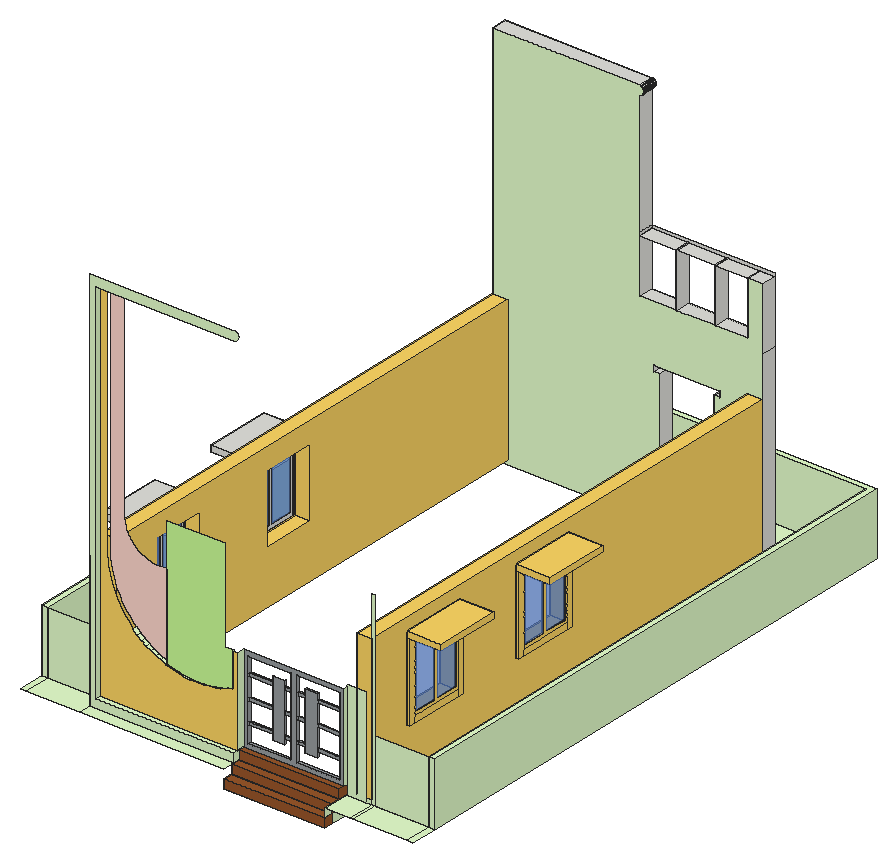
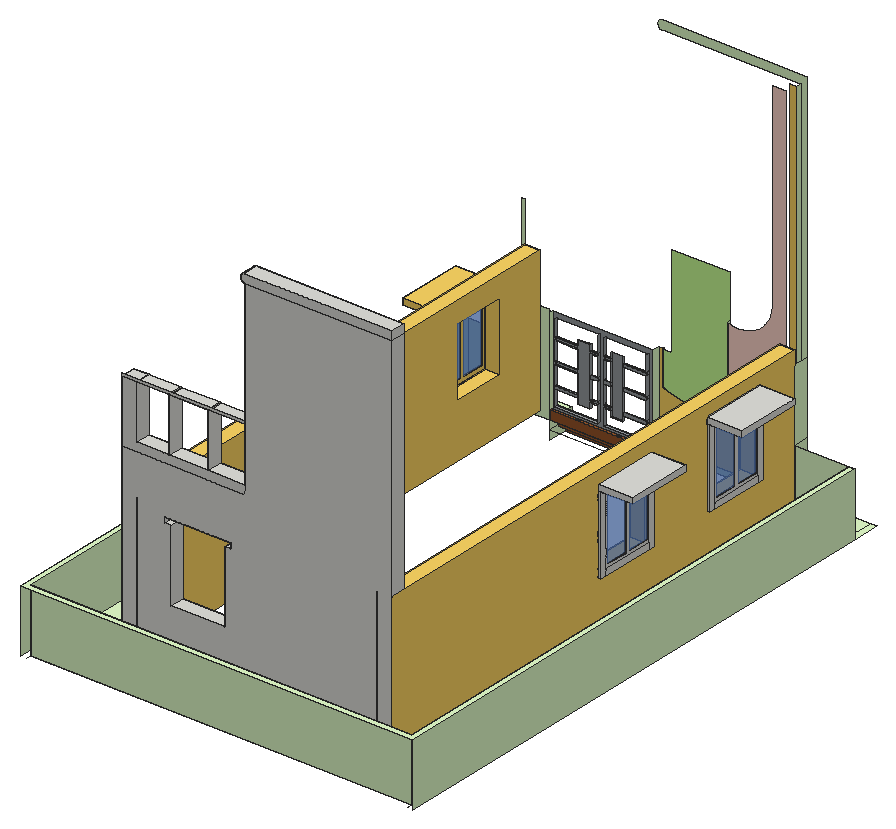
# SketchUp Ruby script. Lengths in inches.
U = 1.inch
M = Sketchup.active_model
def pt(a) = Geom::Point3d.new(a.map { |v| v * U })
def face(e, loops, mat)
  f = e.add_face(loops[0].map { |a| pt(a) })
  loops[1..].each { |l| e.add_face(l.map { |a| pt(a) }).erase! }
  f.material = f.back_material = mat if mat
  f
end
# faces: each face lists its corners as indices into pts; further lists are holes
def faces(e, pts, list, mat = nil) = list.each { |f| face(e, (f[0].is_a?(Array) ? f : [f]).map { |l| l.map { |i| pts[i] } }, mat) }
# xy, xz, yz: faces in a plane at the given z, y or x. An outline is a flat list of corners, or four numbers for a rectangle; further outlines are holes
def ring(l) = l.size == 4 ? [[l[0], l[1]], [l[2], l[1]], [l[2], l[3]], [l[0], l[3]]] : l.each_slice(2).to_a
def flat(e, list, mat, &to3) = list.each { |f| face(e, (f[0].is_a?(Array) ? f : [f]).map { |l| ring(l).map { |u, v| to3.(u, v) } }, mat) }
def xy(e, z, list, mat = nil) = flat(e, list, mat) { |x, y| [x, y, z] }
def xz(e, y, list, mat = nil) = flat(e, list, mat) { |x, z| [x, y, z] }
def yz(e, x, list, mat = nil) = flat(e, list, mat) { |y, z| [x, y, z] }
def lines(e, pts, list) = list.each { |a, b| e.add_line(pt(pts[a]), pt(pts[b])) }
# prism: a flat outline (further loops are holes) pulled along v
def prism(e, loops, v, mat = nil)
  f = face(e, loops, mat); d = Geom::Vector3d.new(v.map { |x| x * U })
  f.pushpull(f.normal.samedirection?(d) ? d.length : -d.length)
end
def box(e, o, s, mat = nil) = prism(e, [[o, [o[0] + s[0], o[1], o[2]], [o[0] + s[0], o[1] + s[1], o[2]], [o[0], o[1] + s[1], o[2]]]], [0, 0, s[2]], mat)
def at(x, y, z, deg = 0) = Geom::Transformation.translation(pt([x, y, z])) * Geom::Transformation.rotation(ORIGIN, Z_AXIS, deg.degrees)
def axes(o, x, y, z) = Geom::Transformation.new([*x, 0, *y, 0, *z, 0, *pt(o).to_a, 1])
def part(name) = M.definitions.add(name)
# library, detail: a bought-in or finely detailed component or shape, given as its bounding box
def library(name, o, s) = part(name).tap { |d| box(d.entities, o, s) }
def detail(e, o, s) = box(e.add_group.entities, o, s)
def put(e, d, t, mat = nil) = e.add_instance(d, t).tap { |i| i.material = mat if mat }
def group(e, t, mat = nil) = e.add_group.tap { |g| g.transformation = t; g.material = mat if mat }.entities
root = M.entities
M.materials.add("[Color B01]").color = [255, 216, 204]
M.materials.add("[Color D03]").color = [255, 216, 101]
M.materials.add("[Color F01]").color = [229, 255, 204]
M.materials.add("[Color F02]").color = [204, 255, 153]
M.materials.add("[Metal Rough]").color = [153, 157, 160]
M.materials.add("[Translucent Glass Blue]").color = [100, 149, 237]
M.materials["[Translucent Glass Blue]"].alpha = 0.5
M.materials.add("[Wood Cherry Original]").color = [152, 86, 42]
c1 = part("Group\#15")
box(c1.entities,[0,0,0],[67,6,6])
c2 = part("Difference\#2")
prism(c2.entities,[[[10,0,96],[10,0,0],[10,336,0],[10,336,96]],[[10,69,82],[10,69,36],[10,33,36],[10,33,82]],[[10,125,36],[10,125,82],[10,161,82],[10,161,36]]],[-10,0,0])
c3 = part("Group\#28")
box(c3.entities,[0,0,0],[0.5,16,22])
c4 = part("Group\#37")
yz(c4.entities,23,[[0,0,4,28],[4,0,40,4]])
p = [[23,40,28],[23,44,28],[23,40,4]]
lines(c4.entities,p,[[0,1],[0,2]])
g1 = group(c4.entities,at(23,4,0))
xz(g1,0,[[-2,0,0,4]])
g2 = group(g1,at(0,0,0))
xy(g2,0,[[-2,0,0,36]])
xy(g2,4,[[-2,0,0,36]])
xz(g2,36,[[-2,0,0,4]])
yz(g2,-2,[[0,0,36,4]])
yz(g2,0,[[0,0,36,4]])
g3 = group(c4.entities,at(23,40,0))
box(g3,[-2,0,0],[2,4,52])
g4 = group(c4.entities,at(23,0,0))
box(g4,[-2,0,0],[2,4,52])
g5 = group(c4.entities,at(22,4,4))
prism(g5,[[[0,0,0],[0,0,48],[0,36,48],[0,36,0]],[[0,35,46],[0,19,46],[0,19,2],[0,35,2]],[[0,1,2],[0,17,2],[0,17,46],[0,1,46]]],[-1,0,0])
put(g5,c3,axes([0,19,2],[-1,0,0],[0,1,0],[0,0,2]),"[Translucent Glass Blue]")
put(g5,c3,axes([-0.23,1,2],[-1,0,0],[0,1,0],[0,0,2]),"[Translucent Glass Blue]")
g6 = group(c4.entities,at(0,0,52))
yz(g6,23,[[0,0,44,4]])
g7 = group(g6,at(0,0,0))
xy(g7,0,[[0,0,23,44]])
xy(g7,4,[[0,0,23,44]])
xz(g7,0,[[0,0,23,4]])
xz(g7,44,[[0,0,23,4]])
yz(g7,0,[[0,0,44,4]])
xy(root,21,[[0,344.07,4,362.07],[4,344.07,40,362.07],[40,344.07,136,352.07],[203,344.07,220,362.07],[220,344.07,222,362.07],
  [222,344.07,258,362.07],[258,344.07,262,362.07],[4,362.07,40,362.07,40,698.07,220,698.07,220,362.07,258,362.07,258,726.37,4,726.37]],"[Color F01]")
xy(root,27,[[44,352.07,136,355.07],[136,360.07,203,362.07]],"[Color F01]")
xy(root,30,[[139,360.07,167.5,362.07],[171.5,360.07,200,362.07]],"[Metal Rough]")
xy(root,37.02,[[154.51,361.07,162.66,362.07],[176.34,361.07,184.49,362.07]],"[Metal Rough]")
xy(root,40.7,[[139,361.07,154.51,362.07],[162.66,361.07,167.5,362.07],[171.5,361.07,176.34,362.07],[184.49,361.07,200,362.07]],"[Metal Rough]")
xy(root,42.7,[[139,361.07,154.51,362.07],[162.66,361.07,167.5,362.07],[171.5,361.07,176.34,362.07],[184.49,361.07,200,362.07]],"[Metal Rough]")
xy(root,55.2,[[139,361.07,154.51,362.07],[162.66,361.07,167.5,362.07],[171.5,361.07,176.34,362.07],[184.49,361.07,200,362.07]],"[Metal Rough]")
xy(root,57.2,[[139,361.07,154.51,362.07],[162.66,361.07,167.5,362.07],[171.5,361.07,176.34,362.07],[184.49,361.07,200,362.07]],"[Metal Rough]")
xy(root,63,[[0,362.07,4,362.07,4,726.37,258,726.37,258,362.07,262,362.07,262,730.07,0,730.07]],"[Color F01]")
xy(root,69.7,[[139,361.07,154.51,362.07],[162.66,361.07,167.5,362.07],[171.5,361.07,176.34,362.07],[184.49,361.07,200,362.07]],"[Metal Rough]")
xy(root,71.7,[[139,361.07,154.51,362.07],[162.66,361.07,167.5,362.07],[171.5,361.07,176.34,362.07],[184.49,361.07,200,362.07]],"[Metal Rough]")
xz(root,352.07,[[40,21,136,21,136,27,44,27,44,273,136,273,136.38,273.02,136.76,273.1,136.95,273.15,137.125,273.22,137.3,273.3,137.47,273.39,137.64,273.49,137.79,273.6,138.09,273.84,138.22,273.98,138.35,274.13,138.46,274.28,138.57,274.44,138.66,274.61,138.74,274.79,138.82,274.96,138.875,275.15,138.92,275.33,138.96,275.52,138.99,275.71,139,275.9,139,276.1,138.99,276.29,138.96,276.48,138.92,276.67,138.875,276.85,138.82,277.04,138.74,277.21,138.66,277.39,138.57,277.56,138.46,277.72,138.35,277.87,138.22,278.02,138.09,278.16,137.79,278.4,137.64,278.51,137.47,278.61,137.3,278.7,137.125,278.78,136.95,278.85,136.76,278.9,136.38,278.98,136,279,40,279]],"[Color F01]")
xz(root,355.07,[[44,27,136,27,136,85.4,133,85.4,133,62.89,129.08,61.43,125.07,60.24,121,59.31,116.87,58.64,112.71,58.24,108.53,58.11,104.36,58.26,100.2,58.67,96.07,59.36,92,60.3,88,61.51,84.6,62.85,81.28,64.39,78.07,66.14,74.97,68.08,72,70.21,69.17,72.52,66.49,75.01,63.97,77.66,61.61,80.45,59.44,83.39,58.14,85.4,57.45,86.46,55.66,89.65,54.07,92.9375,52.6875,96.32,51.52,99.79,50.57,103.32,49.84,106.9,49.33,110.52,49.05,114.16,49,117.82,49,273,44,273]],"[Color D03]")
xz(root,356.07,[[108.53,58.11,112.71,58.24,116.87,58.64,121,59.31,125.07,60.24,129.08,61.43,133,62.89,133,85.4,126.51,85.4,126.51,147,88,147,88,61.51,92,60.3,96.07,59.36,100.2,58.67,104.36,58.26]],"[Color F02]")
xz(root,358.07,[[88,61.51,88,117.88,86.6,117.45,85.18,117.1,83.75,116.85,82.29,116.69,80.83,116.63,79.37,116.66,77.92,116.78,76.47,117,75.04,117.3125,73.64,117.71,72.26,118.2,70.92,118.78,69.62,119.45,68.36,120.19,67.16,121.02,66.01,121.92,64.92,122.9,63.9,123.9375,62.94,125.04,62.06,126.21,61.61,126.88,61.25,127.43,60.53,128.7,59.89,130.01,59.33,131.36,58.87,132.75,58.49,134.16,58.2,135.59,58.01,137.04,57.91,138.5,57.91,139.96,58,141.42,58,270,49,270,49,117.82,49.05,114.16,49.33,110.52,49.84,106.9,50.57,103.32,51.52,99.79,52.6875,96.32,54.07,92.9375,55.66,89.65,57.45,86.46,58.14,85.4,59.44,83.39,61.61,80.45,63.97,77.66,66.49,75.01,69.17,72.52,72,70.21,74.97,68.08,78.07,66.14,81.28,64.39,84.6,62.85]],"[Color B01]")
xz(root,360.07,[[[136,27,203,85.4],[171.5,30,200,82.4],[139,30,167.5,82.4]]],"[Metal Rough]")
xz(root,361.07,[[154.51,37.02,162.66,75.22],[176.34,37.02,184.49,75.22],[139,40.7,154.51,42.7],[162.66,40.7,167.5,42.7],[171.5,40.7,176.34,42.7],
  [184.49,40.7,200,42.7],[139,55.2,154.51,57.2],[162.66,55.2,167.5,57.2],[171.5,55.2,176.34,57.2],[184.49,55.2,200,57.2],
  [139,69.7,154.51,71.7],[162.66,69.7,167.5,71.7],[171.5,69.7,176.34,71.7],[184.49,69.7,200,71.7]],"[Metal Rough]")
xz(root,362.07,[[0,21,4,63],[4,21,40,63],[203,21,216,21,216,87,204.57,87,204.33,86.94,204.21,86.9,204.09,86.85,203.87,86.73,203.77,86.66,203.67,86.58,203.4,86.31,203.33,86.21,203.26,86.1,203.14,85.88,203.02,85.52,203,85.4],[216,21,220,21,220,91.16,219.96,90.87,219.91,90.58,219.83,90.29,219.74,90.01,219.63,89.73,219.5,89.46,219.36,89.2,219.2,88.95,219.02,88.72,218.83,88.49,218.625,88.27,218.41,88.07,218.18,87.89,217.93,87.72,217.68,87.5625,217.42,87.42,217.14,87.3,216.87,87.2,216.58,87.11,216.29,87.05,216,87],[220,21,222,147],
  [222,21,258,63],[258,21,262,63]],"[Color F01]")
xz(root,362.07,[[176.34,37.02,184.49,75.22],[139,40.7,154.51,42.7],[184.49,40.7,200,42.7],[139,55.2,154.51,57.2],[162.66,55.2,167.5,57.2],
  [171.5,55.2,176.34,57.2],[139,69.7,154.51,71.7]],"[Metal Rough]")
xz(root,688.07,[[[40,21,220,21,220,189,210,189,210,153,188.6,153,188.6,189,187.6,189,187.6,153,162.6,153,162.6,189,161.6,189,161.6,153,137.6,153,137.6,273,138.375,273.1,139.1,273.4,139.72,273.88,140.19,274.5,140.49,275.22,140.59,276,140.49,276.77,140.19,277.5,139.72,278.12,139.1,278.59,138.375,278.89,137.6,278.99,137.6,279,40,279],[151.19,63,151.19,111,147.19,111,147.19,115,191.19,115,191.19,111,187.19,111,187.19,63]]],"[Color F01]")
xz(root,726.37,[[4,21,258,63]],"[Color F01]")
yz(root,0,[[362.07,21,730.07,63]],"[Color F01]")
yz(root,4,[[362.07,21,726.37,63]],"[Color F01]")
yz(root,40,[[352.07,21,362.07,63],[352.07,63,362.07,111]],"[Color F01]")
yz(root,44,[[352.07,27,355.07,273]],"[Color F01]")
yz(root,88,[[356.07,61.51,358.07,117.88]],"[Color F01]")
yz(root,133,[[355.07,62.89,356.07,85.4]],"[Color F01]")
yz(root,136,[[352.07,21,362.07,27],[355.07,27,360.07,85.4]],"[Color F01]")
yz(root,139,[[360.07,30,362.07,40.7],[360.07,40.7,361.07,42.7],[360.07,42.7,362.07,55.2],[360.07,55.2,361.07,57.2],[360.07,57.2,362.07,69.7],
  [360.07,69.7,361.07,71.7],[360.07,71.7,362.07,82.4]],"[Metal Rough]")
yz(root,154.51,[[361.07,37.02,362.07,40.7],[361.07,40.7,362.07,42.7],[361.07,42.7,362.07,55.2],[361.07,55.2,362.07,57.2],[361.07,57.2,362.07,69.7],
  [361.07,69.7,362.07,71.7],[361.07,71.7,362.07,75.22]],"[Metal Rough]")
yz(root,162.66,[[361.07,37.02,362.07,40.7],[361.07,40.7,362.07,42.7],[361.07,42.7,362.07,55.2],[361.07,55.2,362.07,57.2],[361.07,57.2,362.07,69.7],
  [361.07,69.7,362.07,71.7],[361.07,71.7,362.07,75.22]],"[Metal Rough]")
yz(root,167.5,[[360.07,30,362.07,40.7],[360.07,40.7,361.07,42.7],[360.07,42.7,362.07,55.2],[360.07,55.2,361.07,57.2],[360.07,57.2,362.07,69.7],
  [360.07,69.7,361.07,71.7],[360.07,71.7,362.07,82.4]],"[Metal Rough]")
yz(root,171.5,[[360.07,30,362.07,40.7],[360.07,40.7,361.07,42.7],[360.07,42.7,362.07,55.2],[360.07,55.2,361.07,57.2],[360.07,57.2,362.07,57.2,362.07,69.7,361.07,69.7,361.07,71.7,360.07,71.7],
  [360.07,71.7,362.07,82.4]],"[Metal Rough]")
yz(root,176.34,[[361.07,37.02,362.07,40.7],[361.07,42.7,362.07,55.2],[361.07,55.2,362.07,57.2],[361.07,57.2,362.07,69.7],[361.07,71.7,362.07,75.22]],"[Metal Rough]")
yz(root,184.49,[[361.07,37.02,362.07,40.7],[361.07,40.7,362.07,42.7],[361.07,42.7,362.07,55.2],[361.07,57.2,362.07,69.7],[361.07,71.7,362.07,75.22]],"[Metal Rough]")
yz(root,200,[[360.07,30,362.07,40.7],[360.07,40.7,361.07,42.7],[360.07,42.7,362.07,55.2],[360.07,55.2,361.07,57.2],[360.07,57.2,362.07,69.7],
  [360.07,69.7,361.07,71.7],[360.07,71.7,362.07,82.4]],"[Metal Rough]")
yz(root,203,[[344.07,9,362.07,15],[344.07,15,362.07,21],[360.07,27,362.07,85.4]],"[Color F01]")
yz(root,258,[[362.07,21,726.37,63]],"[Color F01]")
yz(root,262,[[362.07,21,730.07,63]],"[Color F01]")
p = [[108.53,355.07,58.11],[108.53,356.07,58.11],[104.36,356.07,58.26],[104.36,355.07,58.26],[112.71,355.07,58.24],[112.71,356.07,58.24],
  [116.87,355.07,58.64],[116.87,356.07,58.64],[100.2,356.07,58.67],[100.2,355.07,58.67],[121,355.07,59.31],[121,356.07,59.31],
  [96.07,356.07,59.36],[96.07,355.07,59.36],[125.07,355.07,60.24],[125.07,356.07,60.24],[92,356.07,60.3],[92,355.07,60.3],
  [129.08,355.07,61.43],[129.08,356.07,61.43],[88,356.07,61.51],[88,355.07,61.51],[133,355.07,62.89],[133,356.07,62.89],
  [88,358.07,61.51],[84.6,358.07,62.85],[84.6,355.07,62.85],[81.28,358.07,64.39],[81.28,355.07,64.39],[78.07,358.07,66.14],
  [78.07,355.07,66.14],[74.97,358.07,68.08],[74.97,355.07,68.08],[72,358.07,70.21],[72,355.07,70.21],[69.17,358.07,72.52],
  [69.17,355.07,72.52],[66.49,358.07,75.01],[66.49,355.07,75.01],[220,698.07,21],[220,698.07,120],[136,362.07,21],
  [203,362.07,21],[136,362.07,15],[203,362.07,15],[258,726.37,21],[258,730.07,21],[4,726.37,21],
  [4,730.07,21]]
faces(root,p,[[0,1,2,3],[4,5,1,0],[6,7,5,4],[3,2,8,9],[10,11,7,6],[9,8,12,13],[14,15,11,10],[13,12,16,17],
  [18,19,15,14],[17,16,20,21],[22,23,19,18],[24,25,26,21,20],[25,27,28,26],[27,29,30,28],[29,31,32,30],[31,33,34,32],
  [33,35,36,34],[35,37,38,36]],"[Color F01]")
lines(root,p,[[39,40],[41,42],[43,44],[45,46],[47,48]])
put(root,c1,axes([136,350.07,9],[1,0,0],[0,0,1],[0,-1,0]),"[Wood Cherry Original]")
put(root,c1,axes([136,356.07,15],[1,0,0],[0,0,1],[0,-1,0]),"[Wood Cherry Original]")
put(root,c1,axes([136,362.07,21],[1,0,0],[0,0,1],[0,-1,0]),"[Wood Cherry Original]")
g8 = group(root,at(220,688.07,21))
xy(g8,168,[[-82.4,0,-58.4,10],[-57.4,0,-32.4,10],[-31.4,0,0,10]])
xz(g8,10,[[-58.4,132,-57.4,168],[-32.4,132,-31.4,168],[-82.4,168,0,170]])
yz(g8,-58.4,[[0,132,10,168]])
yz(g8,-57.4,[[0,132,10,168]])
yz(g8,-32.4,[[0,132,10,168]])
yz(g8,-31.4,[[0,132,10,168]])
g9 = group(g8,at(0,0,0))
xy(g9,0,[[-180,0,0,10]])
xy(g9,42,[[-68.81,0,-32.81,10]])
xy(g9,90,[[-72.81,0,-68.81,10],[-32.81,0,-28.81,10]])
xy(g9,94,[[-72.81,0,-28.81,10]])
xy(g9,132,[[-82.4,0,-58.4,10],[-58.4,0,-57.4,10],[-57.4,0,-32.4,10],[-32.4,0,-31.4,10],[-31.4,0,-10,10]])
xy(g9,168,[[-10,0,0,10]])
xy(g9,258,[[-180,0,-82.4,10]])
xz(g9,10,[[-180,0,0,6],[[-180,6,-180,252,-82.4,252,-82.4,126,0,126,0,6],[-68.81,42,-32.81,42,-32.81,90,-28.81,90,-28.81,94,-72.81,94,-72.81,90,-68.81,90]],[-82.4,126,-82.4,132,-10,132,-10,168,0,168,0,126],[-180,252,-180,258,-82.4,258,-82.02,257.98,-81.64,257.9,-81.46,257.85,-81.28,257.78,-81.1,257.7,-80.93,257.61,-80.77,257.51,-80.61,257.4,-80.46,257.28,-80.32,257.16,-80.18,257.02,-79.94,256.72,-79.84,256.56,-79.74,256.39,-79.66,256.21,-79.59,256.04,-79.53,255.85,-79.48,255.67,-79.44,255.48,-79.4,255.1,-79.4,254.9,-79.44,254.52,-79.48,254.33,-79.53,254.15,-79.59,253.96,-79.66,253.79,-79.74,253.61,-79.84,253.44,-79.94,253.28,-80.18,252.98,-80.32,252.84,-80.46,252.72,-80.61,252.6,-80.77,252.49,-80.93,252.39,-81.1,252.3,-81.28,252.22,-81.46,252.15,-81.64,252.1,-82.02,252.02,-82.4,252]])
yz(g9,-180,[[0,0,10,6],[0,6,10,252],[0,252,10,258]])
yz(g9,-82.4,[[0,132,10,168],[0,168,10,170],[0,170,10,252]])
yz(g9,-79.4,[[0,254.9,10,255.1]])
yz(g9,-72.81,[[0,90,10,94]])
yz(g9,-68.81,[[0,42,10,90]])
yz(g9,-32.81,[[0,42,10,90]])
yz(g9,-28.81,[[0,90,10,94]])
yz(g9,-10,[[0,132,10,168]])
yz(g9,0,[[0,0,10,6],[0,6,10,126],[0,126,10,168]])
p = [[-82.21,0,252.01],[-82.4,0,252],[-82.4,10,252],[-82.21,10,252.01],[-82.02,0,252.02],[-82.02,10,252.02],
  [-81.83,0,252.06],[-81.83,10,252.06],[-81.64,0,252.1],[-81.64,10,252.1],[-81.46,0,252.15],[-81.46,10,252.15],
  [-81.28,0,252.22],[-81.28,10,252.22],[-81.1,0,252.3],[-81.1,10,252.3],[-80.93,0,252.39],[-80.93,10,252.39],
  [-80.77,0,252.49],[-80.77,10,252.49],[-80.61,0,252.6],[-80.61,10,252.6],[-80.46,0,252.72],[-80.46,10,252.72],
  [-80.32,0,252.84],[-80.32,10,252.84],[-80.18,0,252.98],[-80.18,10,252.98],[-80.06,0,253.13],[-80.06,10,253.13],
  [-79.94,0,253.28],[-79.94,10,253.28],[-79.84,0,253.44],[-79.84,10,253.44],[-79.74,0,253.61],[-79.74,10,253.61],
  [-79.66,0,253.79],[-79.66,10,253.79],[-79.59,0,253.96],[-79.59,10,253.96],[-79.53,0,254.15],[-79.53,10,254.15],
  [-79.48,0,254.33],[-79.48,10,254.33],[-79.44,0,254.52],[-79.44,10,254.52],[-79.42,0,254.71],[-79.42,10,254.71],
  [-79.4,0,254.9],[-79.4,10,254.9],[-79.42,0,255.29],[-79.4,0,255.1],[-79.4,10,255.1],[-79.42,10,255.29],
  [-79.44,0,255.48],[-79.44,10,255.48],[-79.48,0,255.67],[-79.48,10,255.67],[-79.53,0,255.85],[-79.53,10,255.85],
  [-79.59,0,256.04],[-79.59,10,256.04],[-79.66,0,256.21],[-79.66,10,256.21],[-79.74,0,256.39],[-79.74,10,256.39],
  [-79.84,0,256.56],[-79.84,10,256.56],[-79.94,0,256.72],[-79.94,10,256.72],[-80.06,0,256.87],[-80.06,10,256.87],
  [-80.18,0,257.02],[-80.18,10,257.02],[-80.32,0,257.16],[-80.32,10,257.16],[-80.46,0,257.28],[-80.46,10,257.28],
  [-80.61,0,257.4],[-80.61,10,257.4],[-80.77,0,257.51],[-80.77,10,257.51],[-80.93,0,257.61],[-80.93,10,257.61],
  [-81.1,0,257.7],[-81.1,10,257.7],[-81.28,0,257.78],[-81.28,10,257.78],[-81.64,0,257.9],[-81.46,0,257.85],
  [-81.46,10,257.85],[-81.64,10,257.9],[-82.02,0,257.98],[-81.83,0,257.94],[-81.83,10,257.94],[-82.02,10,257.98],
  [-82.4,0,258],[-82.21,0,257.99],[-82.21,10,257.99],[-82.4,10,258]]
faces(g9,p,[[0,1,2,3],[4,0,3,5],[6,4,5,7],[8,6,7,9],[10,8,9,11],[12,10,11,13],[14,12,13,15],[16,14,15,17],
  [18,16,17,19],[20,18,19,21],[22,20,21,23],[24,22,23,25],[26,24,25,27],[28,26,27,29],[30,28,29,31],[32,30,31,33],
  [34,32,33,35],[36,34,35,37],[38,36,37,39],[40,38,39,41],[42,40,41,43],[44,42,43,45],[46,44,45,47],[48,46,47,49],
  [50,51,52,53],[54,50,53,55],[56,54,55,57],[58,56,57,59],[60,58,59,61],[62,60,61,63],[64,62,63,65],[66,64,65,67],
  [68,66,67,69],[70,68,69,71],[72,70,71,73],[74,72,73,75],[76,74,75,77],[78,76,77,79],[80,78,79,81],[82,80,81,83],
  [84,82,83,85],[86,84,85,87],[88,89,90,91],[89,86,87,90],[92,93,94,95],[93,88,91,94],[96,97,98,99],[97,92,95,98]])
put(root,c2,at(40,362.07,24),"[Color D03]")
g10 = group(root,at(210,362.07,24),"[Color D03]")
put(g10,c4,axes([33,119.82,32],[-1,0,0],[0,1,0],[0,0,1]))
put(g10,c4,axes([33,29.03,32],[-1,0,0],[0,1,0],[0,0,1]))
put(g10,c2,at(0,0,0))
put(root,c4,at(17,391.11,56))
put(root,c4,at(17,481.9,56))
